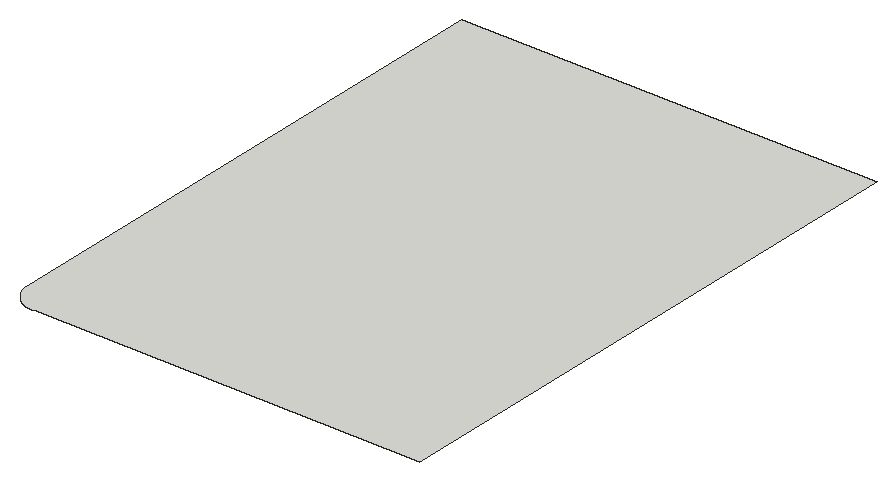
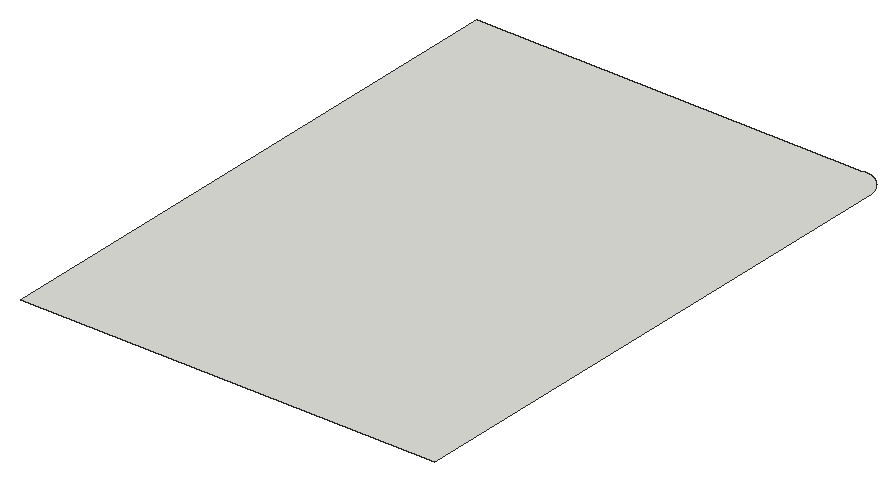
# SketchUp Ruby script. Lengths in inches.
U = 1.inch
M = Sketchup.active_model
def pt(a) = Geom::Point3d.new(a.map { |v| v * U })
def face(e, loops, mat)
  f = e.add_face(loops[0].map { |a| pt(a) })
  loops[1..].each { |l| e.add_face(l.map { |a| pt(a) }).erase! }
  f.material = f.back_material = mat if mat
  f
end
# faces: each face lists its corners as indices into pts; further lists are holes
def faces(e, pts, list, mat = nil) = list.each { |f| face(e, (f[0].is_a?(Array) ? f : [f]).map { |l| l.map { |i| pts[i] } }, mat) }
# xy, xz, yz: faces in a plane at the given z, y or x. An outline is a flat list of corners, or four numbers for a rectangle; further outlines are holes
def ring(l) = l.size == 4 ? [[l[0], l[1]], [l[2], l[1]], [l[2], l[3]], [l[0], l[3]]] : l.each_slice(2).to_a
def flat(e, list, mat, &to3) = list.each { |f| face(e, (f[0].is_a?(Array) ? f : [f]).map { |l| ring(l).map { |u, v| to3.(u, v) } }, mat) }
def xy(e, z, list, mat = nil) = flat(e, list, mat) { |x, y| [x, y, z] }
def xz(e, y, list, mat = nil) = flat(e, list, mat) { |x, z| [x, y, z] }
def yz(e, x, list, mat = nil) = flat(e, list, mat) { |y, z| [x, y, z] }
def lines(e, pts, list) = list.each { |a, b| e.add_line(pt(pts[a]), pt(pts[b])) }
# prism: a flat outline (further loops are holes) pulled along v
def prism(e, loops, v, mat = nil)
  f = face(e, loops, mat); d = Geom::Vector3d.new(v.map { |x| x * U })
  f.pushpull(f.normal.samedirection?(d) ? d.length : -d.length)
end
def box(e, o, s, mat = nil) = prism(e, [[o, [o[0] + s[0], o[1], o[2]], [o[0] + s[0], o[1] + s[1], o[2]], [o[0], o[1] + s[1], o[2]]]], [0, 0, s[2]], mat)
def at(x, y, z, deg = 0) = Geom::Transformation.translation(pt([x, y, z])) * Geom::Transformation.rotation(ORIGIN, Z_AXIS, deg.degrees)
def axes(o, x, y, z) = Geom::Transformation.new([*x, 0, *y, 0, *z, 0, *pt(o).to_a, 1])
def part(name) = M.definitions.add(name)
# library, detail: a bought-in or finely detailed component or shape, given as its bounding box
def library(name, o, s) = part(name).tap { |d| box(d.entities, o, s) }
def detail(e, o, s) = box(e.add_group.entities, o, s)
def put(e, d, t, mat = nil) = e.add_instance(d, t).tap { |i| i.material = mat if mat }
def group(e, t, mat = nil) = e.add_group.tap { |g| g.transformation = t; g.material = mat if mat }.entities
root = M.entities
M.materials.add("1122 AP 7994 PEACH ROSE").color = [254, 227, 201]
xy(root,152.82,[[40.86,180.07,40.7,180.09,40.55,180.11,40.47,180.12,40.39,180.14,40.32,180.15,40.16,180.19,40.09,180.22,40.01,180.24,39.8,180.33,39.72,180.36,39.65,180.4,39.58,180.43,39.52,180.47,39.38,180.55,39.32,180.6,39.25,180.64,38.95,180.89,38.89,180.95,38.84,181.01,38.79,181.0625,38.74,181.12,38.68,181.18,38.64,181.24,38.59,181.31,38.54,181.37,38.5,181.4375,38.46,181.5,38.34,181.71,38.28,181.85,38.24,181.92,38.22,182,38.1875,182.07,38.16,182.14,38.14,182.22,38.12,182.29,38.08,182.45,38.07,182.52,38.05,182.6,38.03,182.76,38.03,182.84,38.02,182.91,38.02,183.23,38.03,183.31,38.03,183.38,38.05,183.54,38.07,183.62,38.08,183.69,38.12,183.85,38.14,183.92,38.16,184,38.1875,184.07,38.22,184.15,38.24,184.22,38.28,184.29,38.34,184.43,38.46,184.64,38.5,184.7,38.54,184.77,38.59,184.83,38.64,184.9,38.68,184.96,38.74,185.02,38.84,185.14,38.95,185.25,39.25,185.5,39.32,185.54,39.38,185.59,39.52,185.67,39.58,185.71,39.65,185.74,39.72,185.78,39.8,185.8125,39.87,185.84,40.01,185.9,40.09,185.92,40.16,185.95,40.32,185.99,40.39,186.01,40.55,186.03,40.625,186.05,40.7,186.05,40.78,186.0625,40.86,186.07,41.17,186.07,41.25,186.0625,41.33,186.05,41.41,186.05,41.49,186.03,41.5625,186.02,41.64,186.01,41.72,185.99,41.79,185.97,41.87,185.95,41.94,185.92,42.02,185.9,42.16,185.84,42.24,185.8125,42.31,185.78,42.38,185.74,42.45,185.71,42.52,185.67,42.58,185.63,42.65,185.59,42.72,185.54,42.78,185.5,43.08,185.25,43.25,185.08,43.4,184.9,43.44,184.83,43.49,184.77,43.53,184.7,43.57,184.64,43.65,184.5,43.6875,184.43,43.72,184.36,43.76,184.29,43.82,184.15,43.84,184.07,43.87,184,43.89,183.92,43.91,183.85,43.95,183.69,43.97,183.62,44,183.38,44.01,183.31,44.01,183.23,44.02,183.15,44.02,182.99,44.01,182.91,44.01,182.84,43.97,182.52,43.95,182.45,43.91,182.29,43.89,182.22,43.87,182.14,43.84,182.07,43.82,182,43.79,181.92,43.76,181.85,43.72,181.78,43.6875,181.71,43.65,181.64,43.57,181.5,43.53,181.4375,43.49,181.37,43.44,181.31,43.4,181.24,43.3,181.12,43.25,181.0625,43.19,181.01,43.14,180.95,43.08,180.89,42.78,180.64,42.72,180.6,42.65,180.55,42.58,180.51,42.52,180.47,42.45,180.43,42.38,180.4,42.31,180.36,42.24,180.33,42.16,180.3,42.02,180.24,41.94,180.22,41.87,180.19,41.79,180.17,41.72,180.15,41.64,180.14,41.5625,180.12,41.49,180.11,41.17,180.07],[104.79,180.07,104.72,180.08,104.4,180.12,104.33,180.14,104.25,180.15,104.17,180.17,104.1,180.19,104.02,180.22,103.95,180.24,103.8,180.3,103.66,180.36,103.59,180.4,103.52,180.43,103.38,180.51,103.32,180.55,103.25,180.6,103.1875,180.64,103,180.79,102.94,180.84,102.83,180.95,102.78,181.01,102.72,181.0625,102.67,181.12,102.57,181.24,102.52,181.31,102.48,181.37,102.44,181.4375,102.39,181.5,102.31,181.64,102.28,181.71,102.24,181.78,102.18,181.92,102.15,182,102.1,182.14,102.07,182.22,102.05,182.29,102.03,182.37,102.02,182.45,102,182.52,101.96,182.84,101.96,182.91,101.95,182.99,101.95,183.15,101.96,183.23,101.96,183.31,101.97,183.38,102,183.62,102.02,183.69,102.03,183.77,102.05,183.85,102.07,183.92,102.1,184,102.125,184.07,102.15,184.15,102.24,184.36,102.28,184.43,102.31,184.5,102.39,184.64,102.44,184.7,102.48,184.77,102.52,184.83,102.57,184.9,102.72,185.08,102.94,185.3,103,185.35,103.1875,185.5,103.25,185.54,103.32,185.59,103.38,185.63,103.52,185.71,103.59,185.74,103.66,185.78,103.73,185.8125,103.8,185.84,103.95,185.9,104.02,185.92,104.1,185.95,104.17,185.97,104.33,186.01,104.4,186.02,104.48,186.03,104.56,186.05,104.64,186.05,104.72,186.0625,104.79,186.07,105.11,186.07,105.1875,186.0625,105.26,186.05,105.34,186.05,105.42,186.03,105.5,186.02,105.57,186.01,105.73,185.97,105.8,185.95,105.88,185.92,105.95,185.9,106.03,185.87,106.1,185.84,106.17,185.8125,106.24,185.78,106.3125,185.74,106.38,185.71,106.59,185.59,106.65,185.54,106.71,185.5,106.78,185.45,107.02,185.25,107.07,185.19,107.13,185.14,107.33,184.9,107.38,184.83,107.42,184.77,107.47,184.7,107.51,184.64,107.59,184.5,107.66,184.36,107.75,184.15,107.78,184.07,107.8,184,107.83,183.92,107.85,183.85,107.89,183.69,107.9,183.62,107.91,183.54,107.93,183.46,107.93,183.38,107.94,183.31,107.95,183.23,107.95,182.91,107.94,182.84,107.93,182.76,107.93,182.68,107.91,182.6,107.9,182.52,107.89,182.45,107.85,182.29,107.83,182.22,107.8,182.14,107.78,182.07,107.75,182,107.72,181.92,107.66,181.78,107.59,181.64,107.51,181.5,107.47,181.4375,107.42,181.37,107.38,181.31,107.33,181.24,107.23,181.12,107.18,181.0625,107.13,181.01,107.07,180.95,107.02,180.89,106.78,180.69,106.71,180.64,106.65,180.6,106.59,180.55,106.38,180.43,106.3125,180.4,106.24,180.36,106.03,180.27,105.95,180.24,105.88,180.22,105.8,180.19,105.73,180.17,105.65,180.15,105.57,180.14,105.5,180.12,105.26,180.09,105.1875,180.08,105.11,180.07]],"1122 AP 7994 PEACH ROSE")
xy(root,158.82,[[32.75,153,366,153,366,645,9,645,9,176.75,9.01,176.5,9.01,176.25,9.02,175.99,9.03,175.74,9.05,175.49,9.0625,175.24,9.08,174.99,9.11,174.74,9.13,174.49,9.16,174.24,9.1875,173.99,9.22,173.74,9.26,173.49,9.3,173.25,9.38,172.75,9.43,172.5,9.47,172.26,9.52,172.01,9.58,171.76,9.63,171.52,9.69,171.28,9.75,171.03,9.82,170.79,9.88,170.55,9.95,170.3,10.02,170.0625,10.1,169.82,10.17,169.58,10.25,169.34,10.33,169.11,10.51,168.63,10.59,168.4,10.69,168.17,10.78,167.93,10.97,167.47,11.07,167.24,11.18,167.01,11.28,166.78,11.39,166.55,11.5,166.33,11.62,166.1,11.73,165.88,11.85,165.66,11.97,165.4375,12.09,165.22,12.22,165,12.34,164.78,12.47,164.57,12.6,164.35,12.74,164.14,12.87,163.93,13.29,163.3,13.4375,163.1,13.58,162.89,13.88,162.49,14.04,162.29,14.19,162.09,14.35,161.9,14.51,161.7,14.83,161.32,15,161.13,15.16,160.94,15.33,160.75,15.5,160.57,15.68,160.39,15.85,160.21,16.21,159.85,16.39,159.68,16.57,159.5,16.75,159.33,16.94,159.16,17.13,159,17.32,158.83,17.7,158.51,17.9,158.35,18.09,158.19,18.29,158.04,18.49,157.88,18.89,157.58,19.1,157.4375,19.3,157.29,19.93,156.87,20.14,156.74,20.35,156.6,20.57,156.47,20.78,156.34,21,156.22,21.22,156.09,21.4375,155.97,21.66,155.85,21.88,155.73,22.1,155.62,22.33,155.5,22.55,155.39,22.78,155.28,23.01,155.18,23.24,155.07,23.47,154.97,23.93,154.78,24.17,154.69,24.4,154.59,24.63,154.51,25.11,154.33,25.34,154.25,25.58,154.17,25.82,154.1,26.0625,154.02,26.3,153.95,26.55,153.88,26.79,153.82,27.03,153.75,27.28,153.69,27.52,153.63,27.76,153.58,28.01,153.52,28.26,153.47,28.5,153.43,28.75,153.38,29.25,153.3,29.49,153.26,29.74,153.22,29.99,153.1875,30.24,153.16,30.49,153.13,30.74,153.11,30.99,153.08,31.24,153.0625,31.49,153.05,31.74,153.03,31.99,153.02,32.25,153.01,32.5,153.01]])
xz(root,180.07,[[104.79,149.82,104.87,152.82],[104.87,149.82,104.95,152.82],[104.95,149.82,105.03,152.82],[105.03,149.82,105.11,152.82]],"1122 AP 7994 PEACH ROSE")
yz(root,44.01,[[183.23,149.82,183.31,152.82]],"1122 AP 7994 PEACH ROSE")
yz(root,44.02,[[183.07,149.82,183.15,152.82]],"1122 AP 7994 PEACH ROSE")
yz(root,101.95,[[182.99,149.82,183.07,152.82],[183.07,149.82,183.15,152.82]],"1122 AP 7994 PEACH ROSE")
yz(root,101.96,[[182.84,149.82,182.91,152.82],[183.23,149.82,183.31,152.82]],"1122 AP 7994 PEACH ROSE")
yz(root,107.93,[[182.68,149.82,182.76,152.82],[183.38,149.82,183.46,152.82]],"1122 AP 7994 PEACH ROSE")
yz(root,107.95,[[182.91,149.82,182.99,152.82],[182.99,149.82,183.07,152.82],[183.07,149.82,183.15,152.82],[183.15,149.82,183.23,152.82]],"1122 AP 7994 PEACH ROSE")
yz(root,161.95,[[182.99,149.82,183.07,152.82],[183.07,149.82,183.15,152.82]],"1122 AP 7994 PEACH ROSE")
yz(root,161.96,[[182.84,149.82,182.91,152.82],[183.23,149.82,183.31,152.82]],"1122 AP 7994 PEACH ROSE")
p = [[104.33,180.14,149.82],[104.25,180.15,149.82],[104.25,180.15,152.82],[104.33,180.14,152.82],[104.4,180.12,149.82],[104.4,180.12,152.82],
  [104.48,180.11,149.82],[104.48,180.11,152.82],[104.56,180.1,149.82],[104.56,180.1,152.82],[104.64,180.09,149.82],[104.64,180.09,152.82],
  [104.72,180.08,149.82],[104.72,180.08,152.82],[104.79,180.07,149.82],[104.79,180.07,152.82],[105.1875,180.08,149.82],[105.11,180.07,149.82],
  [105.11,180.07,152.82],[105.1875,180.08,152.82],[105.26,180.09,149.82],[105.26,180.09,152.82],[105.34,180.1,149.82],[105.34,180.1,152.82],
  [105.42,180.11,149.82],[105.42,180.11,152.82],[105.5,180.12,149.82],[105.5,180.12,152.82],[105.57,180.14,149.82],[105.57,180.14,152.82],
  [105.65,180.15,149.82],[105.65,180.15,152.82],[103.95,180.24,149.82],[103.875,180.27,149.82],[103.875,180.27,152.82],[103.95,180.24,152.82],
  [104.02,180.22,149.82],[104.02,180.22,152.82],[104.1,180.19,149.82],[104.1,180.19,152.82],[104.17,180.17,149.82],[104.17,180.17,152.82],
  [105.73,180.17,149.82],[105.73,180.17,152.82],[105.8,180.19,149.82],[105.8,180.19,152.82],[105.88,180.22,149.82],[105.88,180.22,152.82],
  [105.95,180.24,149.82],[105.95,180.24,152.82],[106.03,180.27,149.82],[106.03,180.27,152.82],[103.73,180.33,149.82],[103.66,180.36,149.82],
  [103.66,180.36,152.82],[103.73,180.33,152.82],[103.8,180.3,149.82],[103.8,180.3,152.82],[106.1,180.3,149.82],[106.1,180.3,152.82],
  [106.17,180.33,149.82],[106.17,180.33,152.82],[106.24,180.36,149.82],[106.24,180.36,152.82],[103.52,180.43,149.82],[103.45,180.47,149.82],
  [103.45,180.47,152.82],[103.52,180.43,152.82],[103.59,180.4,149.82],[103.59,180.4,152.82],[106.3125,180.4,149.82],[106.3125,180.4,152.82],
  [106.38,180.43,149.82],[106.38,180.43,152.82],[106.45,180.47,149.82],[106.45,180.47,152.82],[103.38,180.51,149.82],[103.32,180.55,149.82],
  [103.32,180.55,152.82],[103.38,180.51,152.82],[106.52,180.51,149.82],[106.52,180.51,152.82],[106.59,180.55,149.82],[106.59,180.55,152.82],
  [163.38,180.51,149.82],[163.32,180.55,149.82],[163.32,180.55,152.82],[163.38,180.51,152.82],[163.45,180.47,149.82],[163.45,180.47,152.82],
  [103.1875,180.64,149.82],[103.125,180.69,149.82],[103.125,180.69,152.82],[103.1875,180.64,152.82],[103.25,180.6,149.82],[103.25,180.6,152.82],
  [106.65,180.6,149.82],[106.65,180.6,152.82],[106.71,180.64,149.82],[106.71,180.64,152.82],[106.78,180.69,149.82],[106.78,180.69,152.82],
  [163.1875,180.64,149.82],[163.125,180.69,149.82],[163.125,180.69,152.82],[163.1875,180.64,152.82],[163.25,180.6,149.82],[163.25,180.6,152.82],
  [103.0625,180.74,149.82],[103,180.79,149.82],[103,180.79,152.82],[103.0625,180.74,152.82],[106.84,180.74,149.82],[106.84,180.74,152.82],
  [106.9,180.79,149.82],[106.9,180.79,152.82],[163.0625,180.74,149.82],[163,180.79,149.82],[163,180.79,152.82],[163.0625,180.74,152.82],
  [102.94,180.84,149.82],[102.89,180.89,149.82],[102.89,180.89,152.82],[102.94,180.84,152.82],[106.96,180.84,149.82],[106.96,180.84,152.82],
  [107.02,180.89,149.82],[107.02,180.89,152.82],[162.94,180.84,149.82],[162.89,180.89,149.82],[162.89,180.89,152.82],[162.94,180.84,152.82],
  [102.83,180.95,149.82],[102.78,181.01,149.82],[102.78,181.01,152.82],[102.83,180.95,152.82],[107.07,180.95,149.82],[107.07,180.95,152.82],
  [107.13,181.01,149.82],[107.13,181.01,152.82],[162.83,180.95,149.82],[162.78,181.01,149.82],[162.78,181.01,152.82],[162.83,180.95,152.82],
  [102.72,181.0625,149.82],[102.72,181.0625,152.82],[107.18,181.0625,149.82],[107.18,181.0625,152.82],[162.72,181.0625,149.82],[162.72,181.0625,152.82],
  [102.67,181.12,149.82],[102.62,181.18,149.82],[102.62,181.18,152.82],[102.67,181.12,152.82],[107.23,181.12,149.82],[107.23,181.12,152.82],
  [107.28,181.18,149.82],[107.28,181.18,152.82],[162.67,181.12,149.82],[162.62,181.18,149.82],[162.62,181.18,152.82],[162.67,181.12,152.82],
  [102.57,181.24,149.82],[102.52,181.31,149.82],[102.52,181.31,152.82],[102.57,181.24,152.82],[107.33,181.24,149.82],[107.33,181.24,152.82],
  [107.38,181.31,149.82],[107.38,181.31,152.82],[162.57,181.24,149.82],[162.52,181.31,149.82],[162.52,181.31,152.82],[162.57,181.24,152.82],
  [102.48,181.37,149.82],[102.48,181.37,152.82],[107.42,181.37,149.82],[107.42,181.37,152.82],[162.48,181.37,149.82],[162.48,181.37,152.82],
  [102.44,181.4375,149.82],[102.39,181.5,149.82],[102.39,181.5,152.82],[102.44,181.4375,152.82],[107.47,181.4375,149.82],[107.47,181.4375,152.82],
  [107.51,181.5,149.82],[107.51,181.5,152.82],[162.44,181.4375,149.82],[162.39,181.5,149.82],[162.39,181.5,152.82],[162.44,181.4375,152.82],
  [102.35,181.57,149.82],[102.35,181.57,152.82],[107.55,181.57,149.82],[107.55,181.57,152.82],[162.35,181.57,149.82],[162.35,181.57,152.82],
  [102.31,181.64,149.82],[102.28,181.71,149.82],[102.28,181.71,152.82],[102.31,181.64,152.82],[107.59,181.64,149.82],[107.59,181.64,152.82],
  [107.625,181.71,149.82],[107.625,181.71,152.82],[162.31,181.64,149.82],[162.28,181.71,149.82],[162.28,181.71,152.82],[162.31,181.64,152.82],
  [102.24,181.78,149.82],[102.24,181.78,152.82],[107.66,181.78,149.82],[107.66,181.78,152.82],[162.24,181.78,149.82],[162.24,181.78,152.82],
  [102.21,181.85,149.82],[102.21,181.85,152.82],[107.69,181.85,149.82],[107.69,181.85,152.82],[162.21,181.85,149.82],[162.21,181.85,152.82],
  [102.18,181.92,149.82],[102.15,182,149.82],[102.15,182,152.82],[102.18,181.92,152.82],[107.72,181.92,149.82],[107.72,181.92,152.82],
  [107.75,182,149.82],[107.75,182,152.82],[162.18,181.92,149.82],[162.15,182,149.82],[162.15,182,152.82],[162.18,181.92,152.82],
  [102.125,182.07,149.82],[102.125,182.07,152.82],[107.78,182.07,149.82],[107.78,182.07,152.82],[162.125,182.07,149.82],[162.125,182.07,152.82],
  [102.1,182.14,149.82],[102.07,182.22,149.82],[102.07,182.22,152.82],[102.1,182.14,152.82],[107.8,182.14,149.82],[107.8,182.14,152.82],
  [107.83,182.22,149.82],[107.83,182.22,152.82],[162.1,182.14,149.82],[162.07,182.22,149.82],[162.07,182.22,152.82],[162.1,182.14,152.82],
  [102.05,182.29,149.82],[102.05,182.29,152.82],[107.85,182.29,149.82],[107.85,182.29,152.82],[162.05,182.29,149.82],[162.05,182.29,152.82],
  [102.03,182.37,149.82],[102.03,182.37,152.82],[107.87,182.37,149.82],[107.87,182.37,152.82],[162.03,182.37,149.82],[162.03,182.37,152.82],
  [102.02,182.45,149.82],[102,182.52,149.82],[102,182.52,152.82],[102.02,182.45,152.82],[107.89,182.45,149.82],[107.89,182.45,152.82],
  [107.9,182.52,149.82],[107.9,182.52,152.82],[162.02,182.45,149.82],[162,182.52,149.82],[162,182.52,152.82],[162.02,182.45,152.82],
  [101.99,182.6,149.82],[101.99,182.6,152.82],[107.91,182.6,149.82],[107.91,182.6,152.82],[161.99,182.6,149.82],[161.99,182.6,152.82],
  [101.98,182.68,149.82],[101.98,182.68,152.82],[107.93,182.68,149.82],[107.93,182.68,152.82],[161.98,182.68,149.82],[161.98,182.68,152.82],
  [101.97,182.76,149.82],[101.97,182.76,152.82],[161.97,182.76,149.82],[161.97,182.76,152.82],[101.96,182.84,149.82],[101.96,182.84,152.82],
  [107.94,182.84,149.82],[107.93,182.76,149.82],[107.93,182.76,152.82],[107.94,182.84,152.82],[107.95,182.91,149.82],[107.95,182.91,152.82],
  [161.96,182.84,149.82],[161.96,182.84,152.82],[101.96,182.91,149.82],[101.95,182.99,149.82],[101.95,182.99,152.82],[101.96,182.91,152.82],
  [161.96,182.91,149.82],[161.95,182.99,149.82],[161.95,182.99,152.82],[161.96,182.91,152.82],[44.01,183.23,149.82],[44.02,183.15,149.82],
  [44.02,183.15,152.82],[44.01,183.23,152.82],[101.95,183.15,149.82],[101.96,183.23,149.82],[101.96,183.23,152.82],[101.95,183.15,152.82],
  [161.95,183.15,149.82],[161.96,183.23,149.82],[161.96,183.23,152.82],[161.95,183.15,152.82],[107.94,183.31,149.82],[107.95,183.23,149.82],
  [107.95,183.23,152.82],[107.94,183.31,152.82],[44,183.38,149.82],[44.01,183.31,149.82],[44.01,183.31,152.82],[44,183.38,152.82],
  [101.96,183.31,149.82],[101.97,183.38,149.82],[101.97,183.38,152.82],[101.96,183.31,152.82],[107.93,183.38,149.82],[107.93,183.38,152.82],
  [161.96,183.31,149.82],[161.97,183.38,149.82],[161.97,183.38,152.82],[161.96,183.31,152.82],[43.99,183.46,149.82],[43.99,183.46,152.82],
  [101.98,183.46,149.82],[101.98,183.46,152.82],[161.98,183.46,149.82],[161.98,183.46,152.82],[43.97,183.62,149.82],[43.98,183.54,149.82],
  [43.98,183.54,152.82],[43.97,183.62,152.82],[101.99,183.54,149.82],[101.99,183.54,152.82],[102,183.62,149.82],[102,183.62,152.82],
  [107.9,183.62,149.82],[107.91,183.54,149.82],[107.91,183.54,152.82],[107.9,183.62,152.82],[107.93,183.46,149.82],[107.93,183.46,152.82],
  [161.99,183.54,149.82],[161.99,183.54,152.82],[162,183.62,149.82],[162,183.62,152.82],[43.95,183.69,149.82],[43.95,183.69,152.82],
  [102.02,183.69,149.82],[102.02,183.69,152.82],[107.89,183.69,149.82],[107.89,183.69,152.82],[162.02,183.69,149.82],[162.02,183.69,152.82],
  [43.93,183.77,149.82],[43.93,183.77,152.82],[102.03,183.77,149.82],[102.03,183.77,152.82],[107.87,183.77,149.82],[107.87,183.77,152.82],
  [162.03,183.77,149.82],[162.03,183.77,152.82],[43.89,183.92,149.82],[43.91,183.85,149.82],[43.91,183.85,152.82],[43.89,183.92,152.82],
  [102.05,183.85,149.82],[102.05,183.85,152.82],[102.07,183.92,149.82],[102.07,183.92,152.82],[107.83,183.92,149.82],[107.85,183.85,149.82],
  [107.85,183.85,152.82],[107.83,183.92,152.82],[162.05,183.85,149.82],[162.05,183.85,152.82],[162.07,183.92,149.82],[162.07,183.92,152.82],
  [43.87,184,149.82],[43.87,184,152.82],[102.1,184,149.82],[102.1,184,152.82],[107.8,184,149.82],[107.8,184,152.82],
  [162.1,184,149.82],[162.1,184,152.82],[43.84,184.07,149.82],[43.84,184.07,152.82],[102.125,184.07,149.82],[102.125,184.07,152.82],
  [107.78,184.07,149.82],[107.78,184.07,152.82],[162.125,184.07,149.82],[162.125,184.07,152.82],[43.79,184.22,149.82],[43.82,184.15,149.82],
  [43.82,184.15,152.82],[43.79,184.22,152.82],[102.15,184.15,149.82],[102.15,184.15,152.82],[102.18,184.22,149.82],[102.18,184.22,152.82],
  [107.72,184.22,149.82],[107.75,184.15,149.82],[107.75,184.15,152.82],[107.72,184.22,152.82],[162.15,184.15,149.82],[162.15,184.15,152.82],
  [162.18,184.22,149.82],[162.18,184.22,152.82],[43.76,184.29,149.82],[43.76,184.29,152.82],[102.21,184.29,149.82],[102.21,184.29,152.82],
  [107.69,184.29,149.82],[107.69,184.29,152.82],[162.21,184.29,149.82],[162.21,184.29,152.82],[43.72,184.36,149.82],[43.72,184.36,152.82],
  [102.24,184.36,149.82],[102.24,184.36,152.82],[107.66,184.36,149.82],[107.66,184.36,152.82],[162.24,184.36,149.82],[162.24,184.36,152.82],
  [43.6875,184.43,149.82],[43.6875,184.43,152.82],[102.28,184.43,149.82],[102.28,184.43,152.82],[107.625,184.43,149.82],[107.625,184.43,152.82]]
faces(root,p,[[0,1,2,3],[4,0,3,5],[6,4,5,7],[8,6,7,9],[10,8,9,11],[12,10,11,13],[14,12,13,15],[16,17,18,19],
  [20,16,19,21],[22,20,21,23],[24,22,23,25],[26,24,25,27],[28,26,27,29],[30,28,29,31],[32,33,34,35],[36,32,35,37],
  [38,36,37,39],[40,38,39,41],[1,40,41,2],[42,30,31,43],[44,42,43,45],[46,44,45,47],[48,46,47,49],[50,48,49,51],
  [52,53,54,55],[56,52,55,57],[33,56,57,34],[58,50,51,59],[60,58,59,61],[62,60,61,63],[64,65,66,67],[68,64,67,69],
  [53,68,69,54],[70,62,63,71],[72,70,71,73],[74,72,73,75],[76,77,78,79],[65,76,79,66],[80,74,75,81],[82,80,81,83],
  [84,85,86,87],[88,84,87,89],[90,91,92,93],[94,90,93,95],[77,94,95,78],[96,82,83,97],[98,96,97,99],[100,98,99,101],
  [102,103,104,105],[106,102,105,107],[85,106,107,86],[108,109,110,111],[91,108,111,92],[112,100,101,113],[114,112,113,115],[116,117,118,119],
  [103,116,119,104],[120,121,122,123],[109,120,123,110],[124,114,115,125],[126,124,125,127],[128,129,130,131],[117,128,131,118],[132,133,134,135],
  [121,132,135,122],[136,126,127,137],[138,136,137,139],[140,141,142,143],[129,140,143,130],[133,144,145,134],[146,138,139,147],[141,148,149,142],
  [150,151,152,153],[144,150,153,145],[154,146,147,155],[156,154,155,157],[158,159,160,161],[148,158,161,149],[162,163,164,165],[151,162,165,152],
  [166,156,157,167],[168,166,167,169],[170,171,172,173],[159,170,173,160],[163,174,175,164],[176,168,169,177],[171,178,179,172],[180,181,182,183],
  [174,180,183,175],[184,176,177,185],[186,184,185,187],[188,189,190,191],[178,188,191,179],[181,192,193,182],[194,186,187,195],[189,196,197,190],
  [198,199,200,201],[192,198,201,193],[202,194,195,203],[204,202,203,205],[206,207,208,209],[196,206,209,197],[199,210,211,200],[212,204,205,213],
  [207,214,215,208],[210,216,217,211],[218,212,213,219],[214,220,221,215],[222,223,224,225],[216,222,225,217],[226,218,219,227],[228,226,227,229],
  [230,231,232,233],[220,230,233,221],[223,234,235,224],[236,228,229,237],[231,238,239,232],[240,241,242,243],[234,240,243,235],[244,236,237,245],
  [246,244,245,247],[248,249,250,251],[238,248,251,239],[241,252,253,242],[254,246,247,255],[249,256,257,250],[252,258,259,253],[260,254,255,261],
  [256,262,263,257],[264,265,266,267],[258,264,267,259],[268,260,261,269],[270,268,269,271],[272,273,274,275],[262,272,275,263],[265,276,277,266],
  [278,270,271,279],[273,280,281,274],[276,282,283,277],[284,278,279,285],[280,286,287,281],[282,288,289,283],[286,290,291,287],[288,292,293,289],
  [294,295,296,297],[298,294,297,299],[290,300,301,291],[302,303,304,305],[306,307,308,309],[310,311,312,313],[314,315,316,317],[318,319,320,321],
  [322,323,324,325],[326,327,328,329],[330,331,332,333],[334,322,325,335],[336,337,338,339],[340,326,329,341],[331,342,343,332],[337,344,345,338],
  [346,347,348,349],[347,340,341,348],[342,350,351,343],[350,352,353,351],[354,355,356,357],[355,358,359,356],[344,360,361,345],[360,362,363,361],
  [364,346,349,365],[352,366,367,353],[368,354,357,369],[362,370,371,363],[372,364,365,373],[366,374,375,367],[376,368,369,377],[370,378,379,371],
  [380,381,382,383],[381,372,373,382],[374,384,385,375],[384,386,387,385],[388,389,390,391],[389,376,377,390],[378,392,393,379],[392,394,395,393],
  [396,380,383,397],[386,398,399,387],[400,388,391,401],[394,402,403,395],[404,396,397,405],[398,406,407,399],[408,400,401,409],[402,410,411,403],
  [412,413,414,415],[413,404,405,414],[406,416,417,407],[416,418,419,417],[420,421,422,423],[421,408,409,422],[410,424,425,411],[424,426,427,425],
  [428,412,415,429],[418,430,431,419],[432,420,423,433],[426,434,435,427],[436,428,429,437],[430,438,439,431],[440,432,433,441],[434,442,443,435],
  [444,436,437,445],[438,446,447,439],[448,440,441,449]],"1122 AP 7994 PEACH ROSE")
